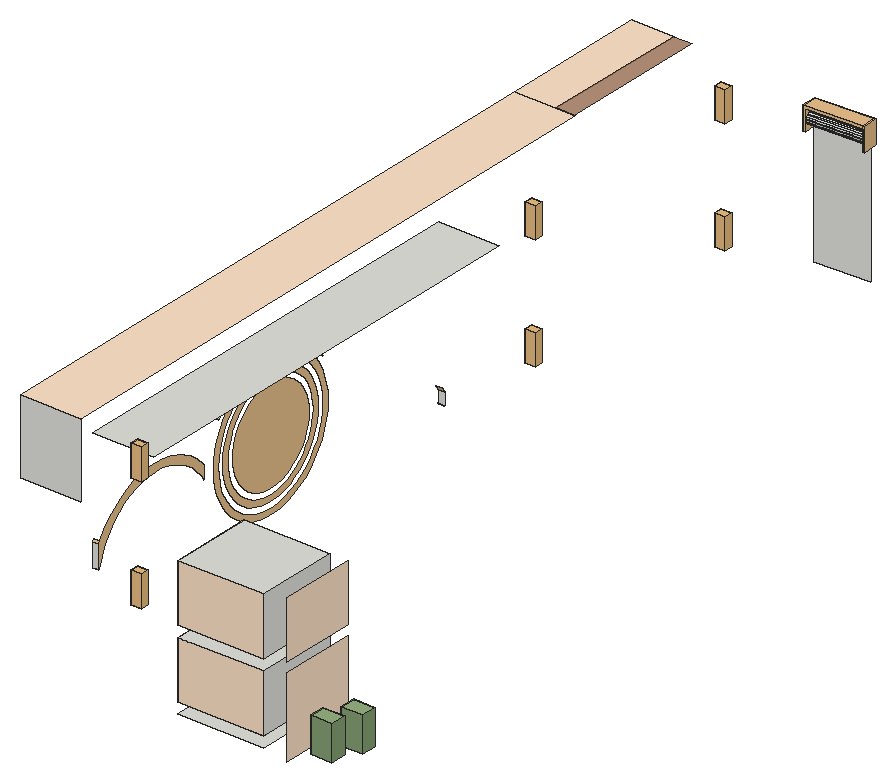
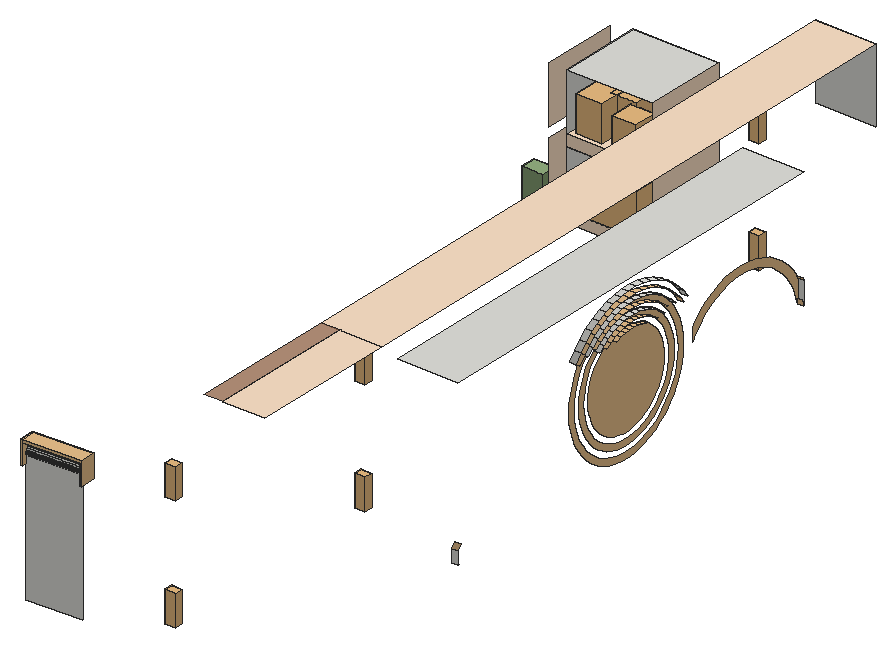
# SketchUp Ruby script. Lengths in inches.
U = 1.inch
M = Sketchup.active_model
def pt(a) = Geom::Point3d.new(a.map { |v| v * U })
def face(e, loops, mat)
  f = e.add_face(loops[0].map { |a| pt(a) })
  loops[1..].each { |l| e.add_face(l.map { |a| pt(a) }).erase! }
  f.material = f.back_material = mat if mat
  f
end
# faces: each face lists its corners as indices into pts; further lists are holes
def faces(e, pts, list, mat = nil) = list.each { |f| face(e, (f[0].is_a?(Array) ? f : [f]).map { |l| l.map { |i| pts[i] } }, mat) }
# xy, xz, yz: faces in a plane at the given z, y or x. An outline is a flat list of corners, or four numbers for a rectangle; further outlines are holes
def ring(l) = l.size == 4 ? [[l[0], l[1]], [l[2], l[1]], [l[2], l[3]], [l[0], l[3]]] : l.each_slice(2).to_a
def flat(e, list, mat, &to3) = list.each { |f| face(e, (f[0].is_a?(Array) ? f : [f]).map { |l| ring(l).map { |u, v| to3.(u, v) } }, mat) }
def xy(e, z, list, mat = nil) = flat(e, list, mat) { |x, y| [x, y, z] }
def xz(e, y, list, mat = nil) = flat(e, list, mat) { |x, z| [x, y, z] }
def yz(e, x, list, mat = nil) = flat(e, list, mat) { |y, z| [x, y, z] }
def lines(e, pts, list) = list.each { |a, b| e.add_line(pt(pts[a]), pt(pts[b])) }
# prism: a flat outline (further loops are holes) pulled along v
def prism(e, loops, v, mat = nil)
  f = face(e, loops, mat); d = Geom::Vector3d.new(v.map { |x| x * U })
  f.pushpull(f.normal.samedirection?(d) ? d.length : -d.length)
end
def box(e, o, s, mat = nil) = prism(e, [[o, [o[0] + s[0], o[1], o[2]], [o[0] + s[0], o[1] + s[1], o[2]], [o[0], o[1] + s[1], o[2]]]], [0, 0, s[2]], mat)
def at(x, y, z, deg = 0) = Geom::Transformation.translation(pt([x, y, z])) * Geom::Transformation.rotation(ORIGIN, Z_AXIS, deg.degrees)
def axes(o, x, y, z) = Geom::Transformation.new([*x, 0, *y, 0, *z, 0, *pt(o).to_a, 1])
def part(name) = M.definitions.add(name)
# library, detail: a bought-in or finely detailed component or shape, given as its bounding box
def library(name, o, s) = part(name).tap { |d| box(d.entities, o, s) }
def detail(e, o, s) = box(e.add_group.entities, o, s)
def put(e, d, t, mat = nil) = e.add_instance(d, t).tap { |i| i.material = mat if mat }
def group(e, t, mat = nil) = e.add_group.tap { |g| g.transformation = t; g.material = mat if mat }.entities
root = M.entities
M.materials.add("QQ截图20130319210408\#1").color = [134, 161, 117]
M.materials.add("QQ截图20130319210422\#1").color = [134, 163, 115]
M.materials.add("QQ截图20130319210439\#1").color = [149, 178, 130]
M.materials.add("[Color C02]").color = [255, 228, 201]
M.materials.add("[Wood Cherry Original]").color = [152, 102, 69]
M.materials["[Wood Cherry Original]"].alpha = 0.74
M.materials.add("images").color = [235, 194, 141]
c1 = library("[SKP_VZ_MOD_01]_WALL_LIGHT",[-1.1,-1.22,0],[3.54,2.36,6.3])
c2 = part("组\#31")
p = [[15.61,0.01,-35.54],[0.01,18.36,-35.54],[0.01,18.36,23.02],[15.61,0.01,23.02],[15.76,0.13,22],[16.02,0.36,21.45],
  [16.38,0.66,21.01],[16.82,1.03,20.7],[17.3,1.44,20.56],[17.79,1.86,20.58],[18.26,2.26,20.76],[18.68,2.62,21.11],
  [19.02,2.9,21.58],[19.25,3.1,22.15],[19.37,3.2,22.78],[19.35,3.18,23.43],[19.21,3.0625,24.05],[18.95,2.84,24.6],
  [18.59,2.54,25.04],[18.15,2.17,25.34],[17.67,1.76,25.49],[17.18,1.34,25.47],[16.71,0.9375,25.28],[16.29,0.58,24.94],
  [15.95,0.29,24.47],[15.72,0.1,23.9],[15.6,0,23.27],[15.62,0.01,22.62],[1.21,19.39,20.7],[1.69,19.8,20.56],
  [2.1875,20.22,20.58],[2.66,20.62,20.76],[0.42,18.71,21.45],[0.16,18.49,22],[0.02,18.37,22.62],[0,18.36,23.27],
  [0.11,18.45,23.9],[0.35,18.65,24.47],[0.68,18.9375,24.94],[1.1,19.3,25.28],[1.57,19.7,25.47],[2.07,20.12,25.49],
  [2.55,20.52,25.34],[2.98,20.89,25.04],[3.34,21.2,24.6],[3.6,21.42,24.05],[3.75,21.54,23.43],[3.76,21.56,22.78],
  [3.65,21.46,22.15],[3.42,21.26,21.58],[3.08,20.97,21.11],[0.78,19.02,21.01],[17.49,1.6,23.02]]
faces(c2.entities,p,[[0,1,2,3],[4,5,6,7,8,9,10,11,12,13,14,15,16,17,18,19,20,21,22,23,24,25,26,3,27],[8,7,28,29],[9,8,29,30],[10,9,30,31],[32,33,34,2,35,36,37,38,39,40,41,42,43,44,45,46,47,48,49,50,31,30,29,28,51],[7,6,51,28],[11,10,31,50],
  [6,5,32,51],[12,11,50,49],[5,4,33,32],[13,12,49,48],[4,27,34,33],[14,13,48,47],[27,3,2,34],[15,14,47,46],
  [3,26,35,2],[26,25,36,35],[16,15,46,45],[25,24,37,36],[17,16,45,44],[24,23,38,37],[18,17,44,43],[23,22,39,38],
  [19,18,43,42],[22,21,40,39],[20,19,42,41],[21,20,41,40]])
lines(c2.entities,p,[[52,3]])
c3 = part("组\#30")
xy(c3.entities,0,[[16.88,0,16.24,0.75,21.43,5.16,22.07,4.41],[0.64,19.11,0,19.86,5.19,24.27,5.83,23.52]])
xy(c3.entities,9.09,[[16.24,0.75,0.64,19.11,5.83,23.52,21.43,5.16]])
xy(c3.entities,10.2,[[16.88,0,22.07,4.41,5.83,23.52,0.64,19.11],[0.64,19.11,5.83,23.52,5.19,24.27,0,19.86]])
p = [[16.24,0.75,0],[16.88,0,0],[16.88,0,10.2],[0.64,19.11,10.2],[0.64,19.11,9.09],[16.24,0.75,9.09],
  [22.07,4.41,0],[22.07,4.41,10.2],[21.43,5.16,9.09],[21.43,5.16,0],[5.83,23.52,9.09],[5.83,23.52,10.2],
  [0,19.86,0],[0.64,19.11,0],[0,19.86,10.2],[5.83,23.52,0],[5.19,24.27,10.2],[5.19,24.27,0]]
faces(c3.entities,p,[[0,1,2,3,4,5],[2,1,6,7],[0,5,8,9],[6,9,8,10,11,7],[12,13,4,3,14],[4,13,15,10],[12,14,16,17],[15,17,16,11,10]])
c4 = library("coffee+cup+lid",[0,0,0.03],[3.7,3.7,4.95])
c5 = library("Group\#224",[-1.61,-1.61,0],[18.66,14.41,13.77])
c6 = part("组\#13")
xy(c6.entities,0,[[0,0,4.33,3.15]],"QQ截图20130319210439\#1")
xy(c6.entities,7.09,[[0,0,4.33,3.15]],"QQ截图20130319210439\#1")
xz(c6.entities,0,[[0,0,4.33,7.09]],"QQ截图20130319210408\#1")
xz(c6.entities,3.15,[[0,0,4.33,7.09]],"QQ截图20130319210408\#1")
yz(c6.entities,0,[[0,0,3.15,7.09]],"QQ截图20130319210422\#1")
yz(c6.entities,4.33,[[0,0,3.15,7.09]],"QQ截图20130319210422\#1")
c7 = part("无标题")
put(c7.entities,c6,at(0,0,0))
xy(root,46.125,[[240.38,11.0625,269.2,38.75]])
xy(root,49.875,[[240.38,11.0625,269.2,38.75]],"[Color C02]")
xy(root,69.1875,[[240.38,11.0625,269.2,38.75]])
xy(root,72.9375,[[240.38,11.0625,269.2,38.75]],"[Color C02]")
xy(root,79.5,[[183.82,117.37,185.82,119.22]],"images")
xy(root,81.5,[[183.82,117.25,185.82,119.34]],"images")
xy(root,85.49,[[183.82,117.03,185.82,119.58]],"images")
xy(root,87.49,[[183.82,116.91,185.82,119.7]])
xy(root,91.48,[[183.82,116.6875,185.82,119.9375]])
xy(root,92.25,[[240.38,11.0625,269.2,38.75]])
xy(root,95.0625,[[183.82,46.5625,204.2,191.0625]])
xy(root,120,[[183.82,16,204.2,222.875],[183.82,222.875,197.82,272]],"[Color C02]")
xy(root,120,[[197.82,222.875,204.2,272]],"[Wood Cherry Original]")
xz(root,11.0625,[[240.38,49.875,269.2,69.1875],[240.38,72.9375,269.2,92.25]],"[Color C02]")
xz(root,16,[[183.82,95.0625,204.2,120]])
xz(root,38.75,[[240.38,46.125,269.2,49.875],[240.38,69.1875,269.2,72.9375]],"[Color C02]")
xz(root,46.5625,[[183.82,54.71,185.82,62.54]])
xz(root,191.0625,[[183.82,40.39,185.82,44.63]])
yz(root,185.82,[[[116.84,39.7,119.625,39.7,122.39,40.02,125.1,40.66,127.72,41.6,130.21,42.85,132.53,44.375,134.67,46.16,136.58,48.18,138.25,50.41,139.64,52.82,140.75,55.375,141.55,58.04,142.04,60.78,142.2,63.56,142.05,66.34,141.57,69.08,140.77,71.75,139.68,74.3,138.29,76.72,136.63,78.95,134.72,80.98,132.59,82.77,130.27,84.3,127.78,85.56,125.17,86.51,122.46,87.16,119.7,87.49,116.91,87.49,114.15,87.17,111.44,86.53,108.82,85.59,106.33,84.34,104.01,82.8125,101.87,81.03,99.96,79.01,98.29,76.78,96.9,74.37,95.79,71.8125,94.99,69.15,94.5,66.41,94.34,63.63,94.49,60.85,94.97,58.11,95.77,55.44,96.87,52.88,98.25,50.47,99.91,48.24,101.82,46.21,103.95,44.42,106.27,42.88,108.76,41.63,111.37,40.68,114.08,40.03],[116.96,41.7,114.43,42,111.95,42.59,109.55,43.47,107.27,44.62,105.15,46.02,103.19,47.66,101.45,49.52,99.93,51.57,98.65,53.78,97.65,56.125,96.92,58.57,96.48,61.08,96.34,63.63,96.49,66.17,96.94,68.68,97.67,71.13,98.68,73.47,99.96,75.67,101.49,77.72,103.24,79.57,105.2,81.21,107.33,82.61,109.61,83.75,112.01,84.62,114.49,85.2,117.03,85.49,119.58,85.49,122.11,85.19,124.59,84.6,126.99,83.72,129.27,82.57,131.4,81.17,133.35,79.53,135.09,77.67,136.61,75.62,137.89,73.41,138.89,71.07,139.62,68.62,140.06,66.11,140.2,63.5625,140.05,61.02,139.61,58.5,138.87,56.0625,137.86,53.72,136.58,51.51,135.05,49.47,133.3,47.62,131.34,45.98,129.21,44.58,126.93,43.44,124.53,42.57,122.05,41.99,119.51,41.7]],[[119.4,43.69,121.7,43.96,123.96,44.49,126.14,45.28,128.21,46.32,130.15,47.59,131.93,49.07,133.52,50.76,134.91,52.62,136.07,54.62,136.99,56.75,137.66,58.97,138.07,61.25,138.2,63.56,138.07,65.88,137.67,68.16,137.01,70.38,136.1,72.51,134.94,74.52,133.56,76.39,131.97,78.07,130.2,79.57,128.26,80.84,126.19,81.89,124.02,82.68,121.76,83.22,119.46,83.49,117.14,83.5,114.84,83.23,112.58,82.7,110.4,81.91,108.33,80.87,106.39,79.6,104.61,78.11,103.02,76.43,101.63,74.57,100.47,72.57,99.55,70.44,98.88,68.22,98.47,65.9375,98.34,63.625,98.47,61.31,98.87,59.03,99.53,56.8,100.44,54.67,101.6,52.67,102.98,50.8,104.57,49.12,106.34,47.62,108.28,46.35,110.35,45.3,112.52,44.51,114.78,43.97,117.08,43.7],[119.29,45.6875,117.2,45.69,115.13,45.9375,113.1,46.42,111.14,47.14,109.28,48.08,107.54,49.23,105.94,50.57,104.51,52.09,103.27,53.76,102.23,55.57,101.41,57.49,100.8125,59.48,100.45,61.54,100.34,63.62,100.46,65.7,100.83,67.76,101.43,69.75,102.26,71.67,103.3,73.47,104.55,75.14,105.98,76.66,107.58,78,109.33,79.14,111.19,80.07,113.15,80.78,115.18,81.26,117.25,81.5,119.34,81.5,121.41,81.25,123.44,80.77,125.4,80.05,127.26,79.11,129,77.96,130.6,76.62,132.03,75.1,133.27,73.43,134.31,71.62,135.13,69.7,135.73,67.7,136.09,65.65,136.2,63.57,136.08,61.49,135.72,59.43,135.11,57.44,134.29,55.52,133.24,53.72,131.99,52.05,130.56,50.53,128.96,49.19,127.21,48.05,125.35,47.12,123.39,46.41,121.36,45.93]],[117.32,47.6875,119.17,47.6875,121.01,47.9,122.82,48.32,124.56,48.95,126.22,49.78,127.77,50.8,129.1875,51.99,130.46,53.33,131.57,54.82,132.5,56.42,133.24,58.12,133.77,59.9,134.09,61.72,134.2,63.57,134.1,65.42,133.78,67.25,133.25,69.02,132.52,70.72,131.6,72.33,130.49,73.82,129.22,75.17,127.81,76.36,126.26,77.38,124.6,78.22,122.86,78.85,121.0625,79.28,119.22,79.5,117.37,79.5,115.53,79.29,113.72,78.87,111.98,78.24,110.32,77.41,108.77,76.39,107.35,75.2,106.08,73.86,104.97,72.37,104.04,70.77,103.31,69.07,102.77,67.29,102.45,65.47,102.34,63.62,102.44,61.77,102.76,59.94,103.29,58.17,104.02,56.46,104.94,54.86,106.05,53.37,107.32,52.02,108.74,50.83,110.28,49.81,111.9375,48.97,113.68,48.34,115.48,47.91],[46.5625,54.71,47.0625,56.78,48.03,59.4,49.3,61.89,50.84,64.21,52.65,66.34,54.68,68.24,56.93,69.9,59.36,71.28,61.92,72.375,64.6,73.16,67.35,73.63,70.14,73.78,72.92,73.61,75.67,73.11,78.34,72.29,80.9,71.18,83.31,69.77,85.54,68.09,87.56,66.17,89.34,64.02,90.41,62.38,90.34,63.64,90.53,66.87,89.56,68.04,87.31,70.18,84.82,72.05,82.14,73.62,79.29,74.86,76.32,75.77,73.26,76.32,70.15,76.52,67.05,76.36,63.98,75.83,61,74.95,58.14,73.74,55.4375,72.19,52.94,70.35,50.66,68.23,48.65,65.86,46.93,63.27,46.5625,62.54]],"images")
yz(root,240.38,[[11.0625,49.875,38.75,69.1875],[11.0625,72.9375,38.75,92.25]],"[Color C02]")
yz(root,269.2,[[11.0625,49.875,38.75,69.1875],[11.0625,72.9375,38.75,92.25]])
yz(root,275.2,[[13.5,42.97,38.75,69.78],[13.5,73.09,38.75,92.25]],"[Color C02]")
p = [[183.82,190.98,40.6],[183.82,191.0625,40.39],[185.82,191.0625,40.39],[185.82,190.98,40.6],[183.82,191.0625,44.63],[183.82,189.95,46.3],
  [185.82,189.95,46.3],[185.82,191.0625,44.63],[183.82,46.5625,54.71],[183.82,47.0625,56.78],[185.82,47.0625,56.78],[185.82,46.5625,54.71],
  [183.82,46.93,63.27],[183.82,46.5625,62.54],[185.82,46.5625,62.54],[185.82,46.93,63.27],[183.82,138.16,80.23],[183.82,139.96,77.8125],
  [185.82,139.96,77.8125],[185.82,138.16,80.23],[183.82,96.625,77.88],[183.82,98.43,80.29],[185.82,98.43,80.29],[185.82,96.625,77.88],
  [183.82,107.58,78],[183.82,109.33,79.14],[185.82,109.33,79.14],[185.82,107.58,78],[183.82,127.26,79.11],[183.82,129,77.96],
  [185.82,129,77.96],[185.82,127.26,79.11],[183.82,106.39,79.6],[183.82,104.61,78.11],[185.82,104.61,78.11],[185.82,106.39,79.6],
  [183.82,131.97,78.07],[183.82,130.2,79.57],[185.82,130.2,79.57],[185.82,131.97,78.07],[183.82,113.72,78.87],[183.82,111.98,78.24],
  [185.82,111.98,78.24],[185.82,113.72,78.87],[183.82,124.6,78.22],[183.82,122.86,78.85],[185.82,122.86,78.85],[185.82,124.6,78.22],
  [183.82,115.53,79.29],[185.82,115.53,79.29],[183.82,121.0625,79.28],[185.82,121.0625,79.28],[183.82,141.63,78.91],[183.82,139.7,81.52],
  [185.82,139.7,81.52],[185.82,141.63,78.91],[183.82,96.9,81.58],[183.82,94.95,78.98],[185.82,94.95,78.98],[185.82,96.9,81.58],
  [183.82,101.87,81.03],[183.82,99.96,79.01],[185.82,99.96,79.01],[185.82,101.87,81.03],[183.82,136.63,78.95],[183.82,134.72,80.98],
  [185.82,134.72,80.98],[185.82,136.63,78.95],[183.82,111.19,80.07],[185.82,111.19,80.07],[183.82,125.4,80.05],[185.82,125.4,80.05],
  [183.82,117.37,79.5],[185.82,117.37,79.5],[183.82,119.22,79.5],[185.82,119.22,79.5],[183.82,131.4,81.17],[183.82,133.35,79.53],
  [185.82,133.35,79.53],[185.82,131.4,81.17],[183.82,103.24,79.57],[183.82,105.2,81.21],[185.82,105.2,81.21],[185.82,103.24,79.57],
  [183.82,108.33,80.87],[185.82,108.33,80.87],[183.82,128.26,80.84],[185.82,128.26,80.84],[183.82,113.15,80.78],[185.82,113.15,80.78],
  [183.82,123.44,80.77],[185.82,123.44,80.77],[183.82,136.1,82.43],[185.82,136.1,82.43],[183.82,100.5,82.49],[185.82,100.5,82.49],
  [183.82,115.18,81.26],[185.82,115.18,81.26],[183.82,121.41,81.25],[185.82,121.41,81.25],[183.82,126.19,81.89],[185.82,126.19,81.89],
  [183.82,110.4,81.91],[185.82,110.4,81.91],[183.82,104.01,82.8125],[185.82,104.01,82.8125],[183.82,132.59,82.77],[185.82,132.59,82.77],
  [183.82,107.33,82.61],[185.82,107.33,82.61],[183.82,129.27,82.57],[185.82,129.27,82.57],[183.82,117.25,81.5],[185.82,117.25,81.5],
  [183.82,119.34,81.5],[185.82,119.34,81.5],[183.82,137.47,83.88],[185.82,137.47,83.88],[183.82,99.13,83.94],[185.82,99.13,83.94],
  [183.82,112.58,82.7],[185.82,112.58,82.7],[183.82,124.02,82.68],[185.82,124.02,82.68],[183.82,133.79,84.375],[185.82,133.79,84.375],
  [183.82,102.81,84.42],[185.82,102.81,84.42],[183.82,109.61,83.75],[185.82,109.61,83.75],[183.82,126.99,83.72],[185.82,126.99,83.72],
  [183.82,114.84,83.23],[185.82,114.84,83.23],[183.82,121.76,83.22],[185.82,121.76,83.22],[183.82,106.33,84.34],[185.82,106.33,84.34],
  [183.82,130.27,84.3],[185.82,130.27,84.3],[183.82,117.14,83.5],[185.82,117.14,83.5],[183.82,119.46,83.49],[185.82,119.46,83.49],
  [183.82,112.01,84.62],[185.82,112.01,84.62],[183.82,124.59,84.6],[185.82,124.59,84.6],[183.82,101.62,86.03],[185.82,101.62,86.03],
  [183.82,134.99,85.98],[185.82,134.99,85.98],[183.82,108.82,85.59],[185.82,108.82,85.59],[183.82,127.78,85.56],[185.82,127.78,85.56],
  [183.82,105.34,86.07],[185.82,105.34,86.07],[183.82,131.27,86.03],[185.82,131.27,86.03],[183.82,114.49,85.2],[185.82,114.49,85.2],
  [183.82,122.11,85.19],[185.82,122.11,85.19],[183.82,117.03,85.49],[185.82,117.03,85.49],[183.82,119.58,85.49],[185.82,119.58,85.49],
  [183.82,111.44,86.53],[185.82,111.44,86.53],[183.82,125.17,86.51],[185.82,125.17,86.51],[183.82,104.34,87.81],[185.82,104.34,87.81],
  [183.82,128.58,87.39],[185.82,128.58,87.39],[183.82,132.27,87.77],[185.82,132.27,87.77],[183.82,108.03,87.42],[185.82,108.03,87.42],
  [183.82,114.15,87.17],[185.82,114.15,87.17],[183.82,122.46,87.16],[185.82,122.46,87.16],[183.82,116.91,87.49],[185.82,116.91,87.49],
  [183.82,119.7,87.49],[185.82,119.7,87.49],[183.82,110.87,88.45],[185.82,110.87,88.45],[183.82,125.75,88.43],[185.82,125.75,88.43],
  [183.82,107.24,89.26],[185.82,107.24,89.26],[183.82,129.375,89.23],[185.82,129.375,89.23],[183.82,122.8125,89.13],[185.82,122.8125,89.13],
  [183.82,113.81,89.14],[185.82,113.81,89.14],[183.82,116.8,89.49],[185.82,116.8,89.49],[183.82,119.82,89.48],[185.82,119.82,89.48],
  [183.82,126.32,90.34],[185.82,126.32,90.34],[183.82,110.3,90.37],[185.82,110.3,90.37],[183.82,123.16,91.1],[185.82,123.16,91.1],
  [183.82,113.46,91.11],[185.82,113.46,91.11],[183.82,116.6875,91.48],[185.82,116.6875,91.48],[183.82,119.9375,91.48],[185.82,119.9375,91.48]]
faces(root,p,[[0,1,2,3],[32,33,34,35],[36,37,38,39],[52,53,54,55],[56,57,58,59],[60,61,62,63],[64,65,66,67],[84,32,35,85],
  [37,86,87,38],[86,100,101,87],[102,84,85,103],[104,60,63,105],[65,106,107,66],[53,116,117,54],[118,56,59,119],[120,102,103,121],
  [100,122,123,101],[132,120,121,133],[122,134,135,123],[136,104,105,137],[106,138,139,107],[140,132,133,141],[134,142,143,135],[142,140,141,143],
  [148,118,119,149],[116,150,151,117],[152,136,137,153],[138,154,155,139],[168,152,153,169],[154,170,171,155],[172,148,149,173],[150,176,177,151],
  [180,168,169,181],[170,182,183,171],[184,180,181,185],[182,186,187,183],[192,172,173,193],[176,194,195,177],[194,204,205,195],[206,192,193,207],
  [204,208,209,205],[210,206,207,211],[212,210,211,213],[208,214,215,209]])
faces(root,p,[[4,5,6,7],[8,9,10,11],[12,13,14,15],[16,17,18,19],[20,21,22,23],[24,25,26,27],[28,29,30,31],[40,41,42,43],
  [44,45,46,47],[48,40,43,49],[45,50,51,46],[25,68,69,26],[70,28,31,71],[72,48,49,73],[50,74,75,51],[76,77,78,79],
  [80,81,82,83],[68,88,89,69],[90,70,71,91],[92,16,19,93],[21,94,95,22],[88,96,97,89],[98,90,91,99],[81,108,109,82],
  [110,76,79,111],[96,112,113,97],[114,98,99,115],[124,92,93,125],[94,126,127,95],[108,128,129,109],[130,110,111,131],[128,144,145,129],
  [146,130,131,147],[126,156,157,127],[158,124,125,159],[144,160,161,145],[162,146,147,163],[160,164,165,161],[166,162,163,167],[174,158,159,175],
  [156,178,179,157],[178,188,189,179],[190,174,175,191],[196,190,191,197],[188,198,199,189],[198,200,201,199],[202,196,197,203],[200,202,203,201]],"images")
put(root,c1,axes([206.7,203.07,55.13],[-1,0,0],[0,-1.15,0],[0,0,1.64]))
put(root,c1,axes([206.7,38.07,55.13],[-1,0,0],[0,-1.15,0],[0,0,1.64]))
put(root,c1,axes([206.7,282.38,55.13],[-1,0,0],[0,-1.15,0],[0,0,1.64]))
put(root,c1,axes([206.7,203.07,93.19],[-1,0,0],[0,-1.15,0],[0,0,1.64]))
put(root,c1,axes([206.7,38.07,93.19],[-1,0,0],[0,-1.15,0],[0,0,1.64]))
put(root,c1,axes([206.7,282.38,93.19],[-1,0,0],[0,-1.15,0],[0,0,1.64]))
g1 = group(root,at(239.26,280.35,53.37))
put(g1,c2,axes([-4.28,22.49,27.01],[-0.46055,-0.60456,0],[0.60456,-0.46055,0],[0,0,0.76]))
put(g1,c3,axes([-4.51,24.52,40.875],[-0.46055,-0.60456,0],[0.60456,-0.46055,0],[0,0,0.76]),"images")
put(root,c4,axes([246.29,30.76,72.87],[2.15985,0,0],[0,2.15985,0],[0,0,2.15985]))
put(root,c5,at(247.43,25.95,49.875))
put(root,c4,axes([252.0625,21.91,72.86],[2.39547,0,0],[0,2.39547,0],[0,0,2.39547]))
put(root,c4,axes([258.8125,28.16,72.86],[2.39547,0,0],[0,2.39547,0],[0,0,2.39547]))
put(root,c7,axes([277.49,20.56,42.97],[1.65,0,0],[0,1.65,0],[0,0,1.65]))
put(root,c7,axes([280.85,29.04,42.97],[1.65,0,0],[0,1.65,0],[0,0,1.65]))
